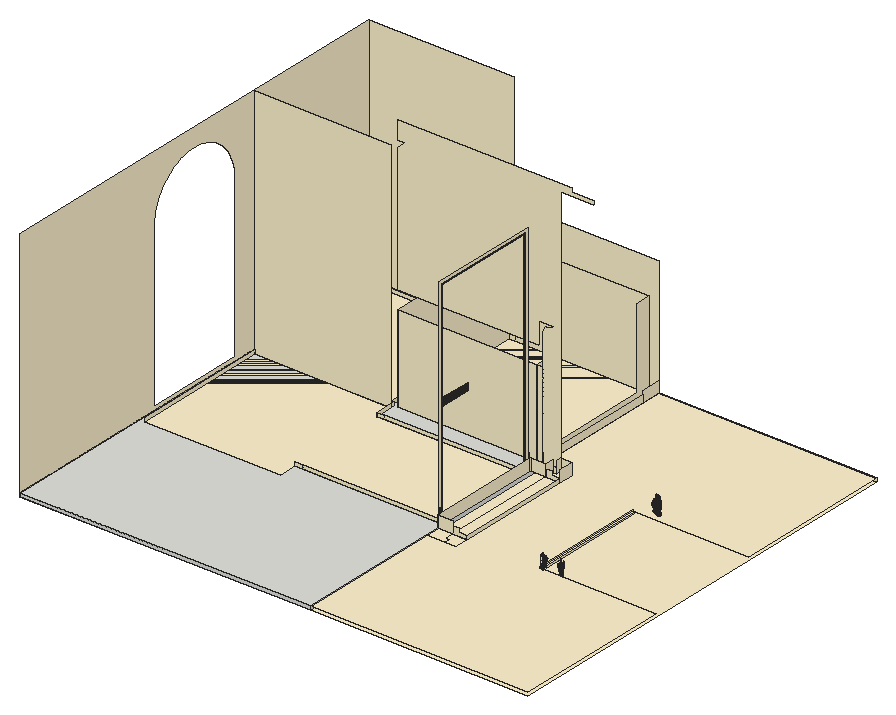
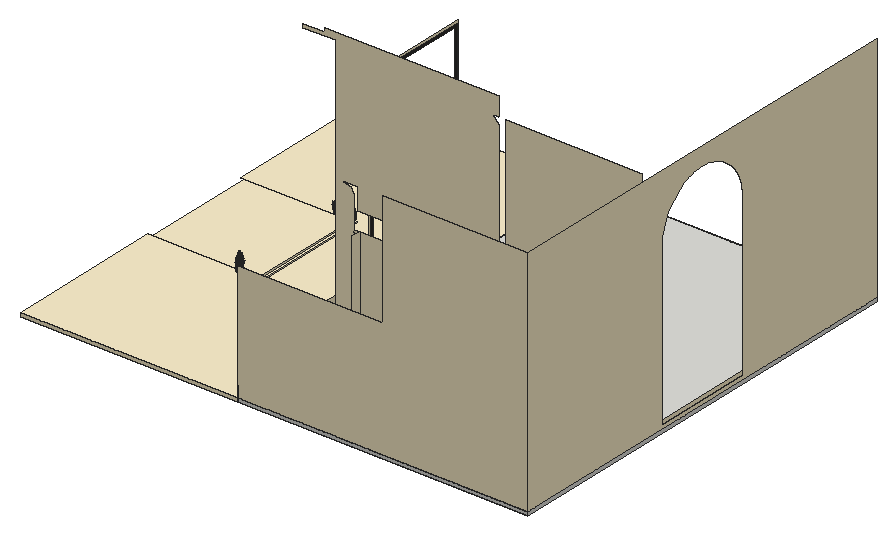
# SketchUp Ruby script. Lengths in inches.
U = 1.inch
M = Sketchup.active_model
def pt(a) = Geom::Point3d.new(a.map { |v| v * U })
def face(e, loops, mat)
  f = e.add_face(loops[0].map { |a| pt(a) })
  loops[1..].each { |l| e.add_face(l.map { |a| pt(a) }).erase! }
  f.material = f.back_material = mat if mat
  f
end
# faces: each face lists its corners as indices into pts; further lists are holes
def faces(e, pts, list, mat = nil) = list.each { |f| face(e, (f[0].is_a?(Array) ? f : [f]).map { |l| l.map { |i| pts[i] } }, mat) }
# xy, xz, yz: faces in a plane at the given z, y or x. An outline is a flat list of corners, or four numbers for a rectangle; further outlines are holes
def ring(l) = l.size == 4 ? [[l[0], l[1]], [l[2], l[1]], [l[2], l[3]], [l[0], l[3]]] : l.each_slice(2).to_a
def flat(e, list, mat, &to3) = list.each { |f| face(e, (f[0].is_a?(Array) ? f : [f]).map { |l| ring(l).map { |u, v| to3.(u, v) } }, mat) }
def xy(e, z, list, mat = nil) = flat(e, list, mat) { |x, y| [x, y, z] }
def xz(e, y, list, mat = nil) = flat(e, list, mat) { |x, z| [x, y, z] }
def yz(e, x, list, mat = nil) = flat(e, list, mat) { |y, z| [x, y, z] }
def lines(e, pts, list) = list.each { |a, b| e.add_line(pt(pts[a]), pt(pts[b])) }
# prism: a flat outline (further loops are holes) pulled along v
def prism(e, loops, v, mat = nil)
  f = face(e, loops, mat); d = Geom::Vector3d.new(v.map { |x| x * U })
  f.pushpull(f.normal.samedirection?(d) ? d.length : -d.length)
end
def box(e, o, s, mat = nil) = prism(e, [[o, [o[0] + s[0], o[1], o[2]], [o[0] + s[0], o[1] + s[1], o[2]], [o[0], o[1] + s[1], o[2]]]], [0, 0, s[2]], mat)
def at(x, y, z, deg = 0) = Geom::Transformation.translation(pt([x, y, z])) * Geom::Transformation.rotation(ORIGIN, Z_AXIS, deg.degrees)
def axes(o, x, y, z) = Geom::Transformation.new([*x, 0, *y, 0, *z, 0, *pt(o).to_a, 1])
def part(name) = M.definitions.add(name)
# library, detail: a bought-in or finely detailed component or shape, given as its bounding box
def library(name, o, s) = part(name).tap { |d| box(d.entities, o, s) }
def detail(e, o, s) = box(e.add_group.entities, o, s)
def put(e, d, t, mat = nil) = e.add_instance(d, t).tap { |i| i.material = mat if mat }
def group(e, t, mat = nil) = e.add_group.tap { |g| g.transformation = t; g.material = mat if mat }.entities
root = M.entities
M.materials.add("D01_Frost_White").color = [255, 242, 206]
M.materials.add("LightPink_Translucent").color = [144, 107, 117]
M.materials["LightPink_Translucent"].alpha = 0.75
M.materials.add("ThomThom - Hat1").color = [48, 46, 44]
c1 = part("blade")
p = [[2.15,0.21,22],[0,0.17,0],[0.09,0.45,0],[2.18,0.31,22],[2.29,0.31,22],[0.38,0.45,0],
  [2.48,0.24,33],[2.49,0.24,33],[2.48,0.22,33]]
faces(c1.entities,p,[[0,1,2,3],[4,5,2,3],[6,3,4,7],[8,0,3,6]])
c2 = part("seeds")
p = [[0.3,-0.1,1.38],[-0.01,-0.03,1.59],[-0.01,-0.03,0.03],[0.14,-0.07,-0.07],[0.29,-0.03,3],[0.15,0.01,3.11]]
faces(c2.entities,p,[[0,1,2,3],[1,0,4,5]],"LightPink_Translucent")
c3 = part("blade with seeds")
put(c3.entities,c1,at(0,0,0))
put(c3.entities,c2,axes([2.4,0.25,30.99],[1.5799,-0.05474,1.17369],[-0.12525,1.92788,0.29478],[-0.07173,-0.02425,1.56792]))
xy(root,-6,[[12,18,492,738]])
xy(root,-6,[[492,18,852,738]],"D01_Frost_White")
xy(root,0,[[12,18,492,738]])
xy(root,0,[[12,18,12,738,252,738,252,498,522,498,522,489,516,489,516,474,491,474,491,470,490,470,490,466,489,466,489,462,246,462,246,498,243,498,243,729,21,729,21,27,243,27,243,258,246,258,246,294,489,294,489,290,490,290,490,286,491,286,491,282,516,282,516,267,522,267,522,258,252,258,252,18],[492,18,852,18,852,282,660.12,282,660.12,474,852,474,852,738,492,738,492,498,540.12,498,540.12,258,492,258],[21,264,21,492,246,492,246,462,489,462,489,294,246,294,246,264],[516,282,540.12,474],[490,286,490,290,489,290,489,466,490,466,490,470,491,470,491,286],
  [21,492,21,729,243,729,243,498,246,498,246,492],[252,498,483,729],[483,498,483,729,252,729,252,738,492,738,492,498]],"D01_Frost_White")
xz(root,18,[[12,-6,492,0]])
xz(root,282,[[491,0,516,19.19],[516,0,516,11.82,526,11.82,526,5.91,540.12,5.91,540.12,0]],"D01_Frost_White")
xz(root,286,[[490,0,491,28]],"D01_Frost_White")
xz(root,290,[[489,0,490,32]],"D01_Frost_White")
xz(root,294,[[246,0,258,6],[258,0,489,6]],"D01_Frost_White")
xz(root,462,[[246,0,258,6],[258,0,486,6],[486,0,489,6]],"D01_Frost_White")
xz(root,466,[[489,0,490,32]],"D01_Frost_White")
xz(root,470,[[490,0,491,28]],"D01_Frost_White")
xz(root,474,[[491,0,516,19.19],[516,0,540.12,0,540.12,5.91,526,5.91,526,11.82,516,11.82]],"D01_Frost_White")
xz(root,489,[[516,0,522,9]],"D01_Frost_White")
xz(root,492,[[21,0,246,390]],"D01_Frost_White")
xz(root,498,[[243,0,246,6],[252,0,483,144],[492,0,492,196,498,205,510,208,510,210,486,210,486,174,252,174,252,384,264,396,252,396,252,426,540,426,540,420,576,420,576,414,522,414,522,0],[483,0,492,144],[522,0,540.12,19.19]],"D01_Frost_White")
xz(root,729,[[21,0,243,6],[252,0,261,144],[261,0,483,144]],"D01_Frost_White")
xz(root,738,[[12,-6,492,0]])
xz(root,738,[[492,-6,852,0],[12,0,12,384,252,384,252,196,492,196,492,0]],"D01_Frost_White")
yz(root,12,[[18,-6,738,0]])
yz(root,12,[[[18,0,738,384],[294,6,462,6,462,275.43,461.51,280.53,460.63,285.98,459.39,291.37,457.8,296.65,455.87,301.83,453.6,306.86,451.01,311.74,448.11,316.43,444.9,320.93,441.41,325.2,437.64,329.24,433.61,333.02,429.35,336.53,424.87,339.75,420.18,342.67,415.3125,345.28,410.29,347.5625,405.12,349.51,399.84,351.12,394.46,352.375,389.01,353.28,383.52,353.82,378,354,372.48,353.82,366.99,353.28,361.54,352.375,356.16,351.12,350.88,349.51,345.71,347.5625,340.6875,345.28,335.82,342.67,331.13,339.75,326.65,336.53,322.39,333.02,318.36,329.24,314.59,325.2,311.1,320.93,307.89,316.43,304.99,311.74,302.4,306.86,300.13,301.83,298.2,296.65,296.61,291.37,295.37,285.98,294.49,280.53,294,275.43]]],"D01_Frost_White")
yz(root,21,[[264,0,492,6],[492,0,729,6]],"D01_Frost_White")
yz(root,243,[[498,0,729,6]],"D01_Frost_White")
yz(root,246,[[462,0,492,6],[492,0,498,6]],"D01_Frost_White")
yz(root,252,[[498,0,729,144]],"D01_Frost_White")
yz(root,483,[[498,0,498,144,513,144,513,12,705,12,705,144,729,144,729,0]],"D01_Frost_White")
yz(root,489,[[294,0,462,6]],"D01_Frost_White")
yz(root,489,[[290,0,294,0,294,174,347.5,174,347.5,186,294,186,294,264,293.8,269.52,293.96,275.04,294,275.43,294,354,462,354,462,275.43,462.04,275.04,462.0625,274.1875,462.2,269.52,462,264,462,0,466,0,466,358,290,358]],"ThomThom - Hat1")
yz(root,490,[[286,0,290,0,290,358,466,358,466,0,470,0,470,362,286,362]],"D01_Frost_White")
yz(root,491,[[282,0,286,19.19],[286,0,470,19.19],[470,0,474,19.19]],"D01_Frost_White")
yz(root,492,[[18,-6,738,0]])
yz(root,492,[[498,0,513,17.4],[513,0,705,12],[705,0,738,17.4]],"D01_Frost_White")
yz(root,516,[[474,0,489,19.19]],"D01_Frost_White")
yz(root,522,[[489,0,498,19.19]],"D01_Frost_White")
yz(root,540.12,[[282,0,474,5.91],[474,0,498,19.19]],"D01_Frost_White")
yz(root,660.12,[[282,0,474,2]],"D01_Frost_White")
yz(root,666.12,[[288,0,468,2]],"D01_Frost_White")
put(root,c3,axes([665.09,278.97,1.9375],[0.08557,-0.11238,0.85688],[0.35897,0.23257,0.06928],[-0.16194,0.14495,0.36631]))
put(root,c3,axes([664.12,279.55,2.36],[-0.01142,0.0647,0.87472],[0.32418,0.22509,-0.13834],[-0.08487,0.10644,0.07015]))
put(root,c3,axes([665.04,280.1,1.3],[0.14502,-0.05158,0.71501],[0.35805,0.15552,-0.15377],[-0.10657,0.13457,0.3057]))
put(root,c3,axes([665.19,279.53,2.37],[-0.32725,-0.22308,0.24001],[0.34753,-0.1924,0.1979],[-0.06036,0.10466,0.49665]))
put(root,c3,axes([665.1875,279.6,2.26],[-0.31095,0.17214,-0.17707],[-0.29435,-0.19656,0.2286],[-0.04479,0.09987,0.4374]))
put(root,c3,axes([664.08,280.21,2.35],[0.05214,-0.01974,0.88692],[0.43092,0.1313,-0.08381],[-0.01013,0.10932,0.15695]))
put(root,c3,axes([665.4,279.42,2.67],[-0.01196,0.30243,-0.3943],[-0.50354,-0.02031,0.04758],[-0.05314,0.12813,0.55778]))
put(root,c3,axes([665.39,280.27,1.38],[-0.01189,-0.19441,0.5743],[0.29719,0.13866,0.42196],[-0.05845,0.09266,0.12649]))
put(root,c3,axes([665.23,279.85,1.68],[0.0101,-0.16879,0.77173],[0.45413,0.08915,0.10664],[-0.03935,0.17989,0.36441]))
put(root,c3,axes([665.5,279.52,2.5],[0.32898,0.21969,-0.2836],[-0.34753,0.1924,-0.21967],[-0.05006,0.11162,0.54264]))
put(root,c3,axes([665.15,279.4,2.7],[0.50507,0.0162,-0.06749],[-0.01381,0.30672,-0.3746],[-0.03508,0.11813,0.56919]))
put(root,c3,axes([665.14,279.85,1.41],[0.41748,-0.0579,0.03254],[0.09598,0.23326,-0.43152],[-0.02647,0.11808,0.3868]))
put(root,c3,axes([665.87,279.21,1.9375],[-0.01125,-0.12549,0.85688],[0.48751,0.08325,0.06928],[-0.03015,0.17883,0.36631]))
put(root,c3,axes([666.22,279.85,2.53],[-0.45283,-0.08548,0.26641],[0.15485,-0.28101,0.21967],[0.02721,0.11051,0.55128]))
put(root,c3,axes([666.1,279.87,2.37],[-0.33863,0.11112,0.03215],[-0.16575,-0.20263,0.2531],[0.0327,0.08932,0.38595]))
put(root,c3,axes([666.17,279.81,0.75],[0.07437,-0.01779,0.88171],[0.44738,0.09793,-0.1347],[0.01308,0.11037,0.15018]))
put(root,c3,axes([666.27,279.91,2.26],[-0.13855,0.25143,-0.17707],[-0.4042,-0.07334,0.2286],[0.03706,0.10123,0.4374]))
put(root,c3,axes([665.98,280.35,2.36],[0.05825,0.05265,0.87472],[0.47011,0.02068,-0.13834],[0.04727,0.11612,0.07015]))
put(root,c3,axes([666.22,279.64,2.53],[0.13855,-0.25143,0.17707],[0.4042,0.07334,-0.2286],[0.03706,0.10123,0.4374]))
put(root,c3,axes([666.31,279.68,2.49],[0.21934,0.26585,-0.35523],[-0.45151,0.14816,0.04287],[0.05129,0.12845,0.5025]))
put(root,c3,axes([666.77,280.54,2.82],[0.31757,-0.18757,-0.03244],[0.29098,0.20543,-0.14708],[0.02049,0.05821,0.48512]))
put(root,c3,axes([666.47,279.73,2.34],[0.45175,0.08196,-0.25549],[-0.15485,0.28101,-0.1979],[0.04142,0.11314,0.48886]))
put(root,c3,axes([666.09,279.75,2.52],[0.44971,-0.15222,-0.0608],[0.221,0.27017,-0.33747],[0.05933,0.11385,0.51278]))
put(root,c3,axes([667.35,279.78,2.37],[-0.45708,0.07503,0.24001],[-0.07933,-0.29434,0.1979],[0.1075,0.08675,0.49665]))
put(root,c3,axes([667.26,279.84,2.37],[-0.20887,0.2077,0.03215],[-0.29744,-0.12092,0.2531],[0.09616,0.06659,0.38595]))
put(root,c3,axes([666.73,279.15,1.9375],[-0.10505,-0.10498,0.85688],[0.48542,-0.08838,0.06928],[0.10971,0.1648,0.36631]))
put(root,c3,axes([667.14,279.37,1.3],[0.00811,-0.10838,0.71501],[0.38755,-0.12106,-0.15377],[0.11964,0.12972,0.3057]))
put(root,c3,axes([668.11,279.9,1.33],[-0.2947,-0.01025,0.5253],[0.19462,-0.21779,0.29003],[0.11642,0.07737,0.41205]))
put(root,c3,axes([667.48,279.6,2.34],[0.45348,-0.07772,-0.25549],[0.07933,0.29434,-0.1979],[0.1218,0.08435,0.48886]))
put(root,c3,axes([696.35,480.8125,3.9375],[0.19062,-0.00741,0.85688],[-0.12645,0.32094,0.06928],[-0.27165,-0.01985,0.36631]))
put(root,c3,axes([696.42,481.38,3.9375],[0.15946,-0.06916,0.85688],[0.13424,0.31957,0.06928],[-0.25033,0.07223,0.36631]))
put(root,c3,axes([695.93,481.92,3.3],[0.15971,0.02684,0.71501],[0.10294,0.27415,-0.15377],[-0.21694,0.05132,0.3057]))
put(root,c3,axes([697.34,481.05,3.67],[0.13063,-0.0473,0.88532],[0.04505,0.33024,0.06928],[-0.28294,0.04382,0.31642]))
put(root,c3,axes([695.9375,481.27,4.36],[-0.07505,0.04245,0.87472],[0.00638,0.31015,-0.13834],[-0.17202,0.04033,0.07015]))
put(root,c3,axes([696.92,480.52,4.49],[-0.45939,-0.00787,-0.35523],[0.03085,-0.3315,0.04287],[-0.19462,-0.03498,0.5025]))
put(root,c3,axes([696.54,480.6,3.3],[0.08973,0.09103,0.71501],[-0.20675,0.24743,-0.15377],[-0.2123,-0.05914,0.3057]))
put(root,c3,axes([697.1,279.91,1.9375],[0.15946,-0.06916,0.85688],[0.13424,0.31957,0.06928],[-0.25033,0.07223,0.36631]))
put(root,c3,axes([696.18,481.09,4.26],[-0.38192,-0.09121,-0.17707],[0.11139,-0.2661,0.2286],[-0.15377,0.0244,0.4374]))
put(root,c3,axes([696.71,480.3,3.9375],[0.1707,0.05633,0.85688],[-0.35326,0.23632,0.06928],[-0.22018,-0.10661,0.36631]))
put(root,c3,axes([696.61,280.45,1.3],[0.15971,0.02684,0.71501],[0.10294,0.27415,-0.15377],[-0.21694,0.05132,0.3057]))
put(root,c3,axes([695.1,481.58,4.35],[0.05865,0.00877,0.88692],[0.18143,0.28888,-0.08381],[-0.12006,0.07582,0.15695]))
put(root,c3,axes([696.4375,481.23,4.34],[-0.1245,0.29741,-0.25549],[-0.42685,-0.10194,-0.1979],[-0.17186,0.02727,0.48886]))
put(root,c3,axes([696.76,480.58,4.34],[-0.3337,0.21658,-0.25549],[-0.29224,-0.22879,-0.1979],[-0.16955,-0.03295,0.48886]))
put(root,c3,axes([696.22,481.21,2.75],[0.01165,0.05153,0.88171],[-0.23495,0.26909,-0.1347],[-0.16689,-0.01356,0.15018]))
put(root,c3,axes([696.29,479.98,4.35],[0.03407,0.03263,0.88692],[-0.16424,0.29331,-0.08381],[-0.16634,0.00212,0.15695]))
put(root,c3,axes([695.59,482.5,3.38],[0.19152,-0.14818,0.5743],[0.07557,0.23459,0.42196],[-0.13841,0.042,0.12649]))
put(root,c3,axes([696.67,479.78,4.36],[-0.09888,-0.00231,0.87472],[-0.3148,0.23079,-0.13834],[-0.16797,-0.04716,0.07015]))
put(root,c3,axes([696.27,481.06,4.37],[0.12984,-0.29812,0.24001],[0.42685,0.10194,0.1979],[-0.16786,0.01792,0.49665]))
put(root,c3,axes([696.42,480.97,4.52],[0.23123,0.29606,-0.0608],[-0.41039,0.14549,-0.33747],[-0.17294,0.03906,0.51278]))
put(root,c3,axes([696.9375,480.36,4.52],[-0.02461,0.33251,-0.0608],[-0.4659,-0.00909,-0.33747],[-0.17944,-0.0231,0.51278]))
put(root,c3,axes([696.64,480.38,4.26],[-0.26148,-0.20471,-0.17707],[0.29857,-0.19378,0.2286],[-0.1517,-0.02948,0.4374]))
put(root,c3,axes([696.23,480.98,4.37],[-0.16879,-0.22293,0.03215],[0.30779,-0.10912,0.2531],[-0.13568,0.02153,0.38595]))
put(root,c3,axes([697.01,481.59,3.9375],[0.11478,-0.10046,0.85688],[0.28982,0.27117,0.06928],[-0.19878,0.12349,0.36631]))
put(root,c3,axes([696.32,481.86,4.26],[-0.40003,0.04673,-0.17707],[-0.10563,-0.26712,0.2286],[-0.11464,0.07175,0.4374]))
put(root,c3,axes([695.78,280.11,2.35],[0.05865,0.00877,0.88692],[0.18143,0.28888,-0.08381],[-0.12006,0.07582,0.15695]))
put(root,c3,axes([696.1,482.65,2.75],[0.06164,0.03267,0.88171],[0.10452,0.30266,-0.1347],[-0.13662,0.06454,0.15018]))
put(root,c3,axes([696.01,480.87,3.38],[0.2934,-0.0234,0.5743],[-0.18611,0.20614,0.42196],[-0.14499,-0.03092,0.12649]))
put(root,c3,axes([696.37,481.8,4.37],[-0.11397,-0.30091,0.24001],[0.44709,-0.05222,0.1979],[-0.13177,0.07077,0.49665]))
put(root,c3,axes([696.6,480.3,4.55],[0.37952,-0.24129,0.26881],[0.32731,0.25625,0.22165],[-0.17806,-0.04451,0.55625]))
put(root,c3,axes([696.28,481.74,4.37],[-0.31549,-0.13751,0.03215],[0.18368,-0.19581,0.2531],[-0.10115,0.06331,0.38595]))
put(root,c3,axes([696.27,281.02,1.38],[0.19152,-0.14818,0.5743],[0.07557,0.23459,0.42196],[-0.13841,0.042,0.12649]))
put(root,c3,axes([696.92,481.84,3.9375],[0.08557,-0.11238,0.85688],[0.35897,0.23257,0.06928],[-0.16194,0.14495,0.36631]))
put(root,c3,axes([697.6875,280.12,1.9375],[0.11478,-0.10046,0.85688],[0.28982,0.27117,0.06928],[-0.19878,0.12349,0.36631]))
put(root,c3,axes([696.99,280.38,2.26],[-0.40003,0.04673,-0.17707],[-0.10563,-0.26712,0.2286],[-0.11464,0.07175,0.4374]))
put(root,c3,axes([696.58,481.06,4.53],[0.38192,0.09121,0.17707],[-0.11139,0.2661,-0.2286],[-0.15377,0.0244,0.4374]))
put(root,c3,axes([696.65,481.89,4.34],[0.11806,0.29854,-0.25549],[-0.44709,0.05222,-0.1979],[-0.12812,0.08019,0.48886]))
put(root,c3,axes([696.78,281.18,0.75],[0.06164,0.03267,0.88171],[0.10452,0.30266,-0.1347],[-0.13662,0.06454,0.15018]))
put(root,c3,axes([696.77,480.3,4.37],[0.02314,-0.24862,0.03215],[0.34943,0.00682,0.2531],[-0.13385,-0.02602,0.38595]))
put(root,c3,axes([695.95,482.42,4.36],[-0.01142,0.0647,0.87472],[0.32418,0.22509,-0.13834],[-0.08487,0.10644,0.07015]))
put(root,c3,axes([697.76,481.67,3.03],[-0.47805,-0.0536,-0.31177],[0.10088,-0.33065,-0.08182],[-0.14266,-0.04007,0.68817]))
put(root,c3,axes([697.85,479.87,4.72],[-0.30671,0.31344,-0.0681],[-0.44417,-0.18058,-0.37797],[-0.1544,-0.08856,0.57432]))
put(root,c3,axes([697.01,480.49,4.53],[0.26148,0.20471,0.17707],[-0.29857,0.19378,-0.2286],[-0.1517,-0.02948,0.4374]))
put(root,c3,axes([697.05,280.33,2.37],[-0.11397,-0.30091,0.24001],[0.44709,-0.05222,0.1979],[-0.13177,0.07077,0.49665]))
put(root,c3,axes([697.71,480.125,4.49],[-0.39186,-0.15803,-0.35523],[0.27849,-0.27693,0.04287],[-0.14198,-0.09436,0.5025]))
put(root,c3,axes([697.53,480.13,4.34],[-0.45348,0.07772,-0.25549],[-0.07933,-0.29434,-0.1979],[-0.1218,-0.08435,0.48886]))
put(root,c3,axes([696.96,280.27,2.37],[-0.31549,-0.13751,0.03215],[0.18368,-0.19581,0.2531],[-0.10115,0.06331,0.38595]))
put(root,c3,axes([697.13,482.3,3.01],[-0.4301,-0.16348,-0.24825],[0.25708,-0.29314,0],[-0.09796,-0.03723,0.78752]))
put(root,c3,axes([696.95,479.86,2.75],[-0.04451,0.04307,0.88171],[-0.44986,0.09286,-0.1347],[-0.10868,-0.08448,0.15018]))
put(root,c3,axes([696.4375,481.67,4.52],[0.4251,0.18028,-0.0608],[-0.24491,0.26108,-0.33747],[-0.1201,0.09075,0.51278]))
put(root,c3,axes([697.6,280.37,1.9375],[0.08557,-0.11238,0.85688],[0.35897,0.23257,0.06928],[-0.16194,0.14495,0.36631]))
put(root,c3,axes([697.4,482.5,3.1875],[-0.28732,0.32763,0],[-0.4807,-0.18271,-0.25804],[-0.10948,-0.04161,0.81856]))
put(root,c3,axes([697.32,280.41,2.34],[0.11806,0.29854,-0.25549],[-0.44709,0.05222,-0.1979],[-0.12812,0.08019,0.48886]))
put(root,c3,axes([695.74,482.46,4.82],[0.40553,0.08728,-0.03244],[-0.12475,0.26862,-0.14708],[-0.06633,0.04078,0.48512]))
put(root,c3,axes([696.625,280.95,2.36],[-0.01142,0.0647,0.87472],[0.32418,0.22509,-0.13834],[-0.08487,0.10644,0.07015]))
put(root,c3,axes([696.64,481.7,4.53],[0.40003,-0.04673,0.17707],[0.10563,0.26712,-0.2286],[-0.11464,0.07175,0.4374]))
put(root,c3,axes([696.87,482.97,3.3],[0.14502,-0.05158,0.71501],[0.35805,0.15552,-0.15377],[-0.10657,0.13457,0.3057]))
put(root,c3,axes([696.67,480.03,3.0625],[-0.13257,0.26698,-0.01946],[-0.40802,-0.08212,-0.08825],[-0.06195,-0.04367,0.29107]))
put(root,c3,axes([697.73,479.125,4.35],[-0.00857,0.03919,0.88692],[-0.42284,0.14223,-0.08381],[-0.12443,-0.0727,0.15695]))
put(root,c3,axes([697.28,479.69,3.3],[-0.02783,0.10696,0.71501],[-0.40683,0.08954,-0.15377],[-0.0951,-0.13825,0.3057]))
put(root,c3,axes([697.41,479.97,3.9375],[0.10505,0.10498,0.85688],[-0.48542,0.08838,0.06928],[-0.10971,-0.1648,0.36631]))
put(root,c3,axes([698.3,481.72,3.33],[-0.46399,0.21707,-0.14548],[-0.30855,-0.30672,-0.25001],[-0.11448,-0.03115,0.79854]))
put(root,c3,axes([697.11,280.2,2.52],[0.4251,0.18028,-0.0608],[-0.24491,0.26108,-0.33747],[-0.1201,0.09075,0.51278]))
put(root,c3,axes([697.02,482.41,4.37],[-0.32725,-0.22308,0.24001],[0.34753,-0.1924,0.1979],[-0.06036,0.10466,0.49665]))
put(root,c3,axes([697.58,479.92,4.26],[-0.07098,-0.26335,-0.17707],[0.40574,-0.06954,0.2286],[-0.10898,-0.07547,0.4374]))
put(root,c3,axes([696.45,481.25,3.1875],[-0.57465,0,0],[0,-0.36542,-0.25804],[0,-0.08323,0.81856]))
put(root,c3,axes([697.25,482.18,3.01],[-0.10795,-0.28489,-0.15489],[0.42874,-0.0809,0.15489],[-0.08643,-0.03285,0.69487]))
put(root,c3,axes([696.9,482.39,4.37],[-0.37765,-0.01523,0.03215],[0.01035,-0.23004,0.2531],[-0.03952,0.08812,0.38595]))
put(root,c3,axes([697.02,482.48,4.26],[-0.31095,0.17214,-0.17707],[-0.29435,-0.19656,0.2286],[-0.04479,0.09987,0.4374]))
put(root,c3,axes([696.41,280.98,2.82],[0.40553,0.08728,-0.03244],[-0.12475,0.26862,-0.14708],[-0.06633,0.04078,0.48512]))
put(root,c3,axes([698.61,481.96,3.03],[-0.30954,0.24575,-0.31177],[-0.38452,-0.22284,-0.08182],[-0.12404,0.0613,0.68817]))
put(root,c3,axes([697.32,280.23,2.53],[0.40003,-0.04673,0.17707],[0.10563,0.26712,-0.2286],[-0.11464,0.07175,0.4374]))
put(root,c3,axes([697.82,480.13,4.53],[0.07098,0.26335,0.17707],[-0.40574,0.06954,-0.2286],[-0.10898,-0.07547,0.4374]))
put(root,c3,axes([695.91,483.09,4.35],[0.05214,-0.01974,0.88692],[0.43092,0.1313,-0.08381],[-0.01013,0.10932,0.15695]))
put(root,c3,axes([697.55,281.5,1.3],[0.14502,-0.05158,0.71501],[0.35805,0.15552,-0.15377],[-0.10657,0.13457,0.3057]))
put(root,c3,axes([696.89,481.15,3.17],[-0.42746,0.27488,0.15378],[-0.42772,-0.27199,-0.18246],[-0.01493,-0.07806,0.82443]))
put(root,c3,axes([698.65,481.91,3.66],[0.39713,0.13184,0.7563],[-0.38905,0.28403,0.29908],[-0.17427,-0.16834,0.63403]))
put(root,c3,axes([697.14,479.52,3.38],[0.23972,0.1138,0.5743],[-0.34912,0.06841,0.42196],[-0.0747,-0.08746,0.12649]))
put(root,c3,axes([698.83,481.82,3.23],[-0.44875,-0.26316,-0.12596],[0.3776,-0.2955,0.27565],[-0.12084,0.03078,0.84108]))
put(root,c3,axes([698.01,481.57,3.11],[-0.27607,-0.27443,-0.2237],[0.41817,-0.19325,0.10766],[-0.08934,-0.03396,0.71822]))
put(root,c3,axes([697.23,482.29,4.67],[-0.01196,0.30243,-0.3943],[-0.50354,-0.02031,0.04758],[-0.05314,0.12813,0.55778]))
put(root,c3,axes([697.22,483.14,3.38],[-0.01189,-0.19441,0.5743],[0.29719,0.13866,0.42196],[-0.05845,0.09266,0.12649]))
put(root,c3,axes([697.7,280.93,2.37],[-0.32725,-0.22308,0.24001],[0.34753,-0.1924,0.1979],[-0.06036,0.10466,0.49665]))
put(root,c3,axes([697.64,479.82,4.55],[0.51193,-0.08404,0.26881],[0.08885,0.32966,0.22165],[-0.1204,-0.09716,0.55625]))
put(root,c3,axes([698.6,481.77,3.11],[-0.49904,0.02018,-0.2237],[-0.04513,-0.33504,0.10766],[-0.08934,0.03396,0.71822]))
put(root,c3,axes([697.58,280.91,2.37],[-0.37765,-0.01523,0.03215],[0.01035,-0.23004,0.2531],[-0.03952,0.08812,0.38595]))
put(root,c3,axes([697.75,479.89,4.37],[0.20887,-0.2077,0.03215],[0.29744,0.12092,0.2531],[-0.09616,-0.06659,0.38595]))
put(root,c3,axes([697.7,281,2.26],[-0.31095,0.17214,-0.17707],[-0.29435,-0.19656,0.2286],[-0.04479,0.09987,0.4374]))
put(root,c3,axes([697.64,482.33,3.24],[0.4301,0.16348,0.24825],[-0.25708,0.29314,0],[-0.09796,-0.03723,0.78752]))
put(root,c3,axes([697.06,482.72,3.68],[0.0101,-0.16879,0.77173],[0.45413,0.08915,0.10664],[-0.03935,0.17989,0.36441]))
put(root,c3,axes([698.05,481.73,3.22],[0.1218,-0.38743,-0.11714],[0.57753,0.06753,0.25635],[-0.10091,-0.0535,0.7822]))
put(root,c3,axes([699.29,280.49,1.03],[-0.30954,0.24575,-0.31177],[-0.38452,-0.22284,-0.08182],[-0.12404,0.0613,0.68817]))
put(root,c3,axes([696.59,281.61,2.35],[0.05214,-0.01974,0.88692],[0.43092,0.1313,-0.08381],[-0.01013,0.10932,0.15695]))
put(root,c3,axes([698.26,481.82,3.31],[-0.08866,0.29179,0.0724],[-0.43315,-0.05065,-0.20674],[-0.07883,-0.02996,0.63372]))
put(root,c3,axes([698.21,479.28,4.36],[-0.07029,-0.04584,0.87472],[-0.46908,0.02906,-0.13834],[-0.07486,-0.10965,0.07015]))
put(root,c3,axes([699.12,482.63,3.01],[-0.4301,0.16348,-0.24825],[-0.25708,-0.29314,0],[-0.09796,0.03723,0.78752]))
put(root,c3,axes([696.58,481,3.01],[0,-0.32696,-0.24825],[0.51416,0,0],[0,-0.07447,0.78752]))
put(root,c3,axes([696.8,481.31,3.24],[0,0.32696,0.24825],[-0.51416,0,0],[0,-0.07447,0.78752]))
put(root,c3,axes([699.15,482.54,3.1],[-0.28374,-0.32877,-0.02571],[0.4807,-0.18271,0.25804],[-0.11845,0.0313,0.81815]))
put(root,c3,axes([697.91,280.82,2.67],[-0.01196,0.30243,-0.3943],[-0.50354,-0.02031,0.04758],[-0.05314,0.12813,0.55778]))
put(root,c3,axes([697.33,482.39,4.5],[0.32898,0.21969,-0.2836],[-0.34753,0.1924,-0.21967],[-0.05006,0.11162,0.54264]))
put(root,c3,axes([699.02,482.5,3.01],[-0.42874,-0.0809,-0.15489],[0.10795,-0.28489,0.15489],[-0.08643,0.03285,0.69487]))
put(root,c3,axes([697.18,482.23,4.53],[0.31095,-0.17214,0.17707],[0.29435,0.19656,-0.2286],[-0.04479,0.09987,0.4374]))
put(root,c3,axes([697.9,281.67,1.38],[-0.01189,-0.19441,0.5743],[0.29719,0.13866,0.42196],[-0.05845,0.09266,0.12649]))
put(root,c3,axes([697.92,481.38,3.33],[-0.51755,-0.15601,-0.14548],[0.2492,-0.32927,-0.25001],[-0.01626,-0.08084,0.79854]))
put(root,c3,axes([699.27,481.28,3.42],[-0.01255,-0.30784,0.70636],[0.56816,0.0798,0.29908],[-0.13438,0.16845,0.66675]))
put(root,c3,axes([696.99,482.28,4.7],[0.50507,0.0162,-0.06749],[-0.01381,0.30672,-0.3746],[-0.03508,0.11813,0.56919]))
put(root,c3,axes([696.97,482.72,3.41],[0.41748,-0.0579,0.03254],[0.09598,0.23326,-0.43152],[-0.02647,0.11808,0.3868]))
put(root,c3,axes([698.95,481.68,3.33],[0.05355,0.37308,-0.14548],[-0.55775,0.02256,-0.25001],[-0.09822,0.04969,0.79854]))
put(root,c3,axes([697.74,281.25,1.68],[0.0101,-0.16879,0.77173],[0.45413,0.08915,0.10664],[-0.03935,0.17989,0.36441]))
put(root,c3,axes([697.6875,481.05,3.05],[-0.18873,-0.33528,-0.34918],[0.54365,-0.12075,-0.09164],[-0.02086,-0.11353,0.77075]))
